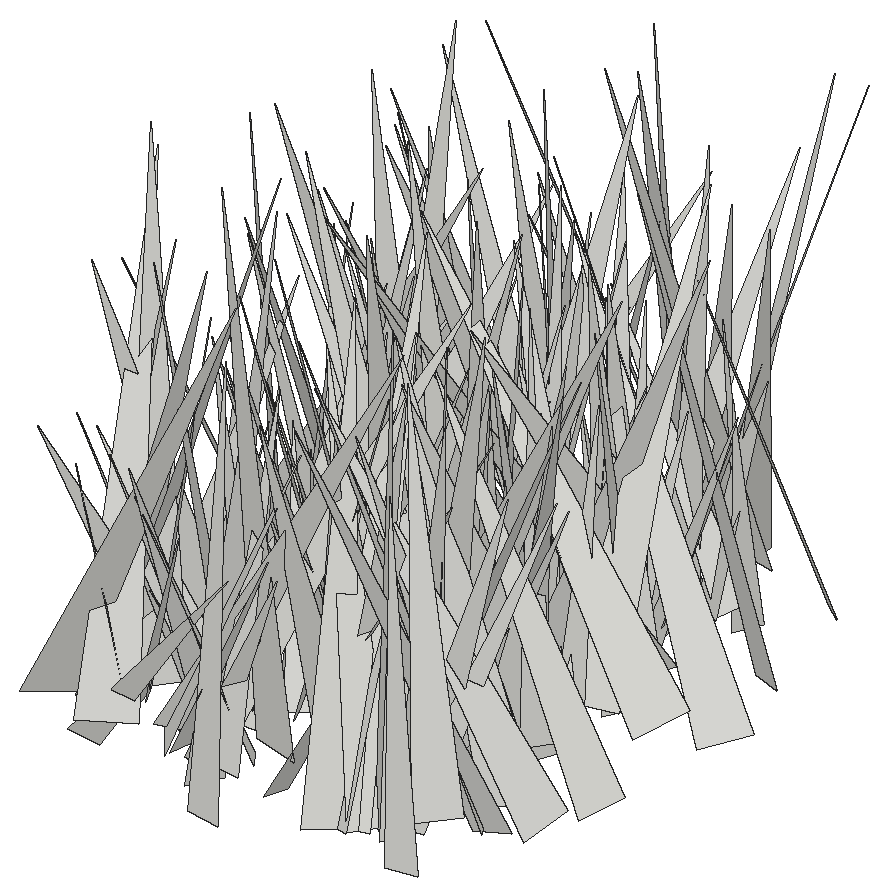
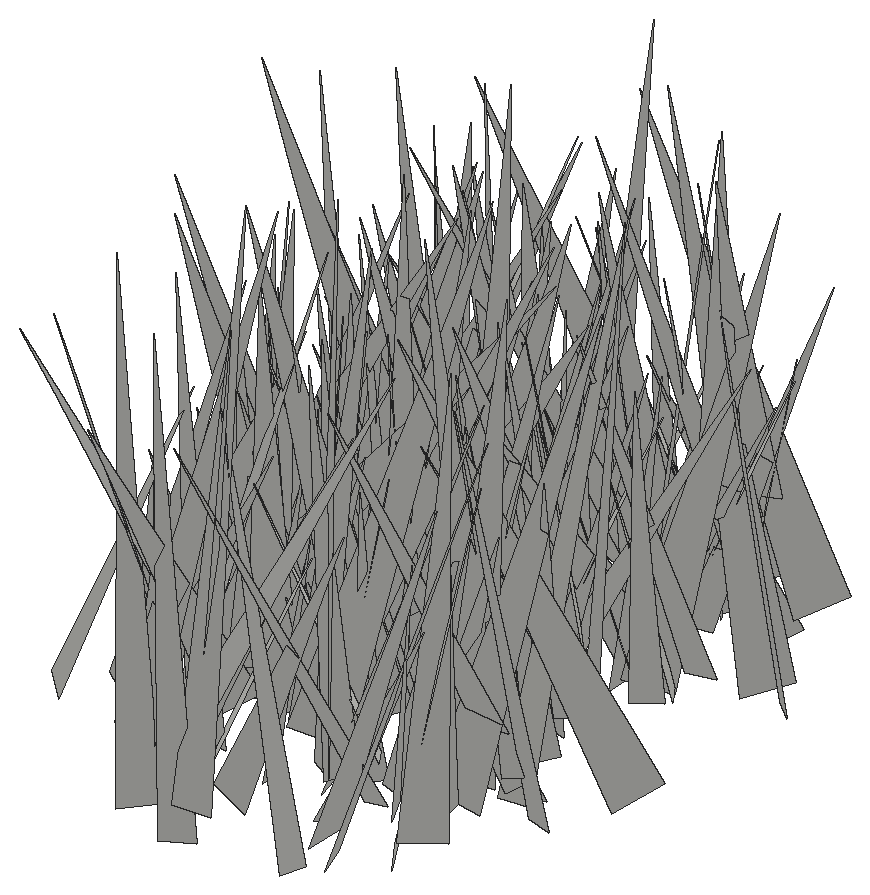
# SketchUp Ruby script. Lengths in inches.
U = 1.inch
M = Sketchup.active_model
def pt(a) = Geom::Point3d.new(a.map { |v| v * U })
def face(e, loops, mat)
  f = e.add_face(loops[0].map { |a| pt(a) })
  loops[1..].each { |l| e.add_face(l.map { |a| pt(a) }).erase! }
  f.material = f.back_material = mat if mat
  f
end
# faces: each face lists its corners as indices into pts; further lists are holes
def faces(e, pts, list, mat = nil) = list.each { |f| face(e, (f[0].is_a?(Array) ? f : [f]).map { |l| l.map { |i| pts[i] } }, mat) }
# xy, xz, yz: faces in a plane at the given z, y or x. An outline is a flat list of corners, or four numbers for a rectangle; further outlines are holes
def ring(l) = l.size == 4 ? [[l[0], l[1]], [l[2], l[1]], [l[2], l[3]], [l[0], l[3]]] : l.each_slice(2).to_a
def flat(e, list, mat, &to3) = list.each { |f| face(e, (f[0].is_a?(Array) ? f : [f]).map { |l| ring(l).map { |u, v| to3.(u, v) } }, mat) }
def xy(e, z, list, mat = nil) = flat(e, list, mat) { |x, y| [x, y, z] }
def xz(e, y, list, mat = nil) = flat(e, list, mat) { |x, z| [x, y, z] }
def yz(e, x, list, mat = nil) = flat(e, list, mat) { |y, z| [x, y, z] }
def lines(e, pts, list) = list.each { |a, b| e.add_line(pt(pts[a]), pt(pts[b])) }
# prism: a flat outline (further loops are holes) pulled along v
def prism(e, loops, v, mat = nil)
  f = face(e, loops, mat); d = Geom::Vector3d.new(v.map { |x| x * U })
  f.pushpull(f.normal.samedirection?(d) ? d.length : -d.length)
end
def box(e, o, s, mat = nil) = prism(e, [[o, [o[0] + s[0], o[1], o[2]], [o[0] + s[0], o[1] + s[1], o[2]], [o[0], o[1] + s[1], o[2]]]], [0, 0, s[2]], mat)
def at(x, y, z, deg = 0) = Geom::Transformation.translation(pt([x, y, z])) * Geom::Transformation.rotation(ORIGIN, Z_AXIS, deg.degrees)
def axes(o, x, y, z) = Geom::Transformation.new([*x, 0, *y, 0, *z, 0, *pt(o).to_a, 1])
def part(name) = M.definitions.add(name)
# library, detail: a bought-in or finely detailed component or shape, given as its bounding box
def library(name, o, s) = part(name).tap { |d| box(d.entities, o, s) }
def detail(e, o, s) = box(e.add_group.entities, o, s)
def put(e, d, t, mat = nil) = e.add_instance(d, t).tap { |i| i.material = mat if mat }
def group(e, t, mat = nil) = e.add_group.tap { |g| g.transformation = t; g.material = mat if mat }.entities
root = M.entities
c1 = part("fur_instance\#9")
p = [[0.8125,0,1.79],[0.67,-0.02,1.48],[0,-0.11,0],[0,0.11,0]]
faces(c1.entities,p,[[0,1,2,3]])
put(root,c1,axes([110.54,92.22,-28.22],[5.37674,4.78999,2.15375],[5.23773,-5.117,-1.69543],[-0.38579,-2.71372,6.99849]))
put(root,c1,axes([113.62,104.89,-28.22],[-4.7875,-3.33897,1.34753],[-3.4677,4.87923,-0.23006],[0.96934,0.96392,5.83232]))
put(root,c1,axes([114.25,101.53,-28.22],[0.14854,-7.36709,1.66817],[-7.40985,-0.46607,-1.39849],[-1.46661,1.60862,7.23466]))
put(root,c1,axes([112.35,95.74,-27.1],[2.0816,-3.74764,1.04429],[-3.88491,-2.06538,0.3318],[-0.20701,1.076,4.27408]))
put(root,c1,axes([111.72,101.13,-28.22],[3.01267,4.99828,1.819],[5.31773,-2.78497,-1.15474],[0.11548,-2.15148,5.72063]))
put(root,c1,axes([114.11,88.5,-27.1],[-5.29033,5.65073,1.03717],[5.57546,5.38985,-0.92613],[1.38587,-0.11308,7.68509]))
put(root,c1,axes([116.16,95.35,-28.22],[-3.99389,-5.07881,0.29207],[-4.86869,3.70838,-2.09153],[-1.47493,1.51142,6.11318]))
put(root,c1,axes([114.78,106.07,-28.22],[-6.09562,-2.74651,0.83103],[-2.67616,6.14538,0.68045],[1.03541,-0.28555,6.65108]))
put(root,c1,axes([114.16,93.5,-28.22],[3.31279,-6.01066,2.01721],[-5.81791,-3.7865,-1.72802],[-2.51972,0.84034,6.64203]))
put(root,c1,axes([112.27,105.35,-27.1],[4.76035,-4.27512,0.72339],[-4.20428,-4.81383,-0.78223],[-1.06017,-0.10597,6.35025]))
put(root,c1,axes([115.68,105.08,-28.22],[-6.67851,0.63047,0.27765],[0.60623,6.66388,-0.54986],[0.32721,0.52189,6.68563]))
put(root,c1,axes([113.89,90.8,-27.1],[5.91163,-3.56463,4.13587],[-4.286,-6.80601,0.26026],[-3.38262,2.39395,6.89828]))
put(root,c1,axes([114.8,91.125,-27.1],[-3.58425,-2.16039,0.18109],[-2.16614,3.55434,-0.47063],[-0.08907,0.49634,4.15845]))
put(root,c1,axes([113.89,104.45,-27.1],[-3.72029,-1.54775,1.40082],[-1.82397,3.80239,-0.64288],[1.01535,1.15959,3.97778]))
put(root,c1,axes([113.86,91.77,-27.1],[3.91388,-2.85851,1.41513],[-2.09693,-3.9939,-2.26798],[-2.40345,-1.17037,4.2832]))
put(root,c1,axes([113.86,89.69,-27.1],[2.36967,1.89121,2.13493],[2.35412,-2.86396,-0.07595],[-1.61018,-1.40392,3.03088]))
put(root,c1,axes([112.15,93.71,-27.1],[0.82135,5.31818,1.14764],[5.3338,-0.55827,-1.23031],[1.07271,-1.29616,5.2387]))
put(root,c1,axes([114.93,96.82,-28.22],[-0.43332,5.55714,0.38235],[5.39105,0.32188,1.43136],[-1.40165,-0.47995,5.3871]))
put(root,c1,axes([115.21,92.45,-28.22],[-4.40105,0.97982,0.44244],[1.06612,4.21791,1.26401],[0.13855,-1.33202,4.328]))
put(root,c1,axes([110.55,98.36,-28.22],[6.56364,-3.25708,1.01889],[-3.38805,-5.95385,2.79299],[0.40967,2.94467,6.77415]))
put(root,c1,axes([114.24,95.81,-28.22],[-4.94486,-5.49387,2.91837],[-6.02867,5.15162,-0.51692],[1.53451,2.53562,7.37341]))
put(root,c1,axes([113.36,93.34,-28.22],[2.95559,2.2846,0.71516],[2.24296,-3.03986,0.44126],[-0.83663,-0.07885,3.70947]))
put(root,c1,axes([112.98,100.57,-28.22],[-2.73458,-7.67612,0.26637],[-7.34259,2.69559,2.30041],[2.25392,-0.53168,7.81722]))
put(root,c1,axes([112.49,101.03,-27.1],[0.76926,-4.66703,1.07076],[-4.59745,-0.41678,1.48633],[1.33832,1.25083,4.49041]))
put(root,c1,axes([111.45,97.96,-28.22],[2.70061,4.81345,0.08968],[4.52857,-2.505,-1.92033],[1.63383,-1.01307,5.17446]))
put(root,c1,axes([114.73,100.41,-28.22],[1.15068,-6.84996,3.27998],[-7.48842,-1.57649,-0.66528],[-1.26644,3.09791,6.914]))
put(root,c1,axes([114.79,93.77,-28.22],[-4.88413,-0.13594,1.40409],[-0.16648,5.08029,-0.08723],[1.4008,0.12978,4.88524]))
put(root,c1,axes([113.99,102.03,-28.22],[3.8396,0.83392,1.68617],[0.96833,-4.16197,-0.14664],[-1.61273,-0.51356,3.92638]))
put(root,c1,axes([114.99,100.08,-28.22],[-4.38014,-2.49103,0.91186],[-2.44951,4.47381,0.4553],[1.01814,0.04674,5.01832]))
put(root,c1,axes([111.52,91.66,-28.22],[8.0282,-2.33719,0.44231],[-2.30718,-8.02996,-0.55383],[-0.57877,-0.40914,8.34313]))
put(root,c1,axes([114.03,90.35,-27.1],[4.42151,2.80893,1.55928],[2.73673,-4.68252,0.67492],[-1.68278,-0.23477,5.19464]))
put(root,c1,axes([116.12,104.46,-28.22],[-3.16167,2.60611,0.16715],[2.5519,3.02748,1.0668],[-0.55458,-0.92652,3.956]))
put(root,c1,axes([112.67,90.4,-27.1],[7.43833,2.19546,1.23858],[2.06036,-7.51855,0.95355],[-1.45225,0.57818,7.69672]))
put(root,c1,axes([115.7,100.08,-27.1],[-3.05082,2.35934,0.28628],[2.37608,3.01778,0.45074],[-0.05159,-0.53147,3.83025]))
put(root,c1,axes([116.54,94.38,-27.1],[-4.07706,-2.14403,0.24298],[-2.12817,3.90987,-1.20919],[-0.35608,1.18084,4.44491]))
put(root,c1,axes([115.99,99.75,-28.22],[-4.01169,-3.78695,1.3287],[-4.00574,3.89344,-0.9976],[0.2459,1.64323,5.42581]))
put(root,c1,axes([115.84,90.8125,-27.1],[-3.47734,-1.80435,0.22841],[-1.8088,3.48242,-0.02761],[0.19,0.12974,3.9175]))
put(root,c1,axes([114.99,94.75,-28.22],[4.45887,4.52554,1.75159],[4.30275,-4.78695,1.41478],[-2.24387,-0.18639,6.19358]))
put(root,c1,axes([112.76,100.27,-28.22],[0.65701,6.39206,0.99008],[6.12037,-0.29236,-2.17392],[2.09278,-1.15171,6.04683]))
put(root,c1,axes([114.97,100.19,-27.1],[-4.71927,-1.33587,1.95814],[-1.09743,5.09822,0.83318],[2.10107,-0.33763,4.83341]))
put(root,c1,axes([113.78,98.33,-28.22],[3.6262,-2.26105,0.60128],[-2.31235,-3.63241,0.28605],[-0.35624,0.56255,4.26378]))
put(root,c1,axes([114.69,99.76,-27.1],[0.76042,7.54721,2.45249],[7.93568,-0.724,-0.23253],[-0.00259,-2.46349,7.58186]))
put(root,c1,axes([111.92,88.86,-27.1],[6.68383,-3.60485,0.36068],[-3.59385,-6.50181,1.61538],[0.45749,1.59067,7.42019]))
put(root,c1,axes([116.02,95.29,-28.22],[-1.82389,-4.57282,0.8897],[-4.65371,1.74485,-0.5721],[-0.21262,1.03617,4.88978]))
put(root,c1,axes([113.45,97.68,-27.1],[0.14432,-5.01914,1.5992],[-4.96199,0.40759,1.72702],[1.76858,1.55311,4.71487]))
put(root,c1,axes([115.32,92.33,-28.22],[-6.01698,-4.0059,2.23214],[-3.85326,6.41302,1.12219],[2.48637,0.24439,7.14087]))
put(root,c1,axes([117.45,102.66,-28.22],[-6.60705,-1.5953,0.55499],[-1.61141,6.62494,-0.14037],[0.50631,0.26714,6.79547]))
put(root,c1,axes([115.55,92.09,-28.22],[-4.95607,3.58078,0.35964],[3.00453,4.45388,-2.94106],[1.98095,2.2034,5.36049]))
put(root,c1,axes([117.55,94.45,-27.1],[-2.16703,-5.16397,2.37315],[-5.48971,1.24499,-2.30381],[-1.47021,2.96275,5.10441]))
put(root,c1,axes([116.35,99.25,-28.22],[-6.49711,1.14641,2.18071],[1.63194,6.61021,1.38712],[1.84567,-1.80917,6.45001]))
put(root,c1,axes([115.87,102.11,-28.22],[-1.28236,-4.10189,0.60594],[-4.14572,1.27987,-0.10961],[0.07509,0.61118,4.29626]))
put(root,c1,axes([112.89,89.08,-28.22],[2.58418,-3.37784,0.00054],[-2.92311,-2.23595,2.1316],[1.69269,1.29557,3.68023]))
put(root,c1,axes([114.99,98.35,-28.22],[2.68413,-2.59886,0.79499],[-2.66781,-2.73276,0.07385],[-0.51851,0.60713,3.7354]))
put(root,c1,axes([114.16,89.83,-27.1],[3.91302,0.34843,0.25725],[0.41449,-3.69091,-1.30566],[-0.12562,-1.32482,3.70519]))
put(root,c1,axes([115.92,90.53,-27.1],[0.4513,-4.46287,0.47479],[-4.46772,-0.49211,-0.3789],[-0.42669,0.43236,4.4696]))
put(root,c1,axes([115.26,98.74,-27.1],[2.93725,2.51058,1.33666],[2.80043,-2.8887,-0.72813],[-0.49727,-1.43859,3.79478]))
put(root,c1,axes([117.31,95.83,-27.1],[2.82941,3.82153,3.56935],[4.50896,-3.83832,0.53527],[-2.64833,-2.45217,4.72474]))
put(root,c1,axes([115.95,96.2,-27.1],[2.7326,-2.75522,2.01665],[-3.2693,-2.85632,0.52755],[-0.98478,1.83723,3.84448]))
put(root,c1,axes([115.56,99.15,-27.1],[2.99735,3.72962,0.28981],[3.68324,-3.00724,0.60693],[-0.65404,0.15682,4.74613]))
put(root,c1,axes([116.83,89.17,-28.22],[-7.30658,0.78889,2.52937],[0.00726,7.42557,-2.29501],[2.64953,2.15518,6.98151]))
put(root,c1,axes([116.79,93.56,-27.1],[-6.46453,1.71895,1.7422],[0.79023,6.12289,-3.109],[2.31637,2.70842,5.92275]))
put(root,c1,axes([118.99,105.15,-28.22],[-0.49335,5.1966,1.87912],[5.02115,-0.36617,2.33091],[-2.30734,-1.90798,4.67065]))
put(root,c1,axes([116.36,96.8,-27.1],[4.45017,0.43948,1.54669],[0.28501,-4.6951,0.51402],[-1.58245,0.39027,4.44218]))
put(root,c1,axes([118.32,89.36,-27.1],[-3.2308,-2.41105,0.08917],[-2.40238,3.20101,-0.49122],[-0.22293,0.4467,4.00124]))
put(root,c1,axes([117.72,92.03,-27.1],[-2.46678,3.0111,0.36551],[3.02886,2.4705,0.08915],[0.1623,-0.33942,3.8915]))
put(root,c1,axes([117.37,92.78,-27.1],[1.88548,3.67223,0.79609],[3.49899,-2.04056,1.12569],[-1.36969,-0.15771,3.97154]))
put(root,c1,axes([115.9,91.76,-27.1],[-0.80392,-5.00028,1.94874],[-5.12712,1.2977,1.21465],[1.58527,1.66129,4.91668]))
put(root,c1,axes([114.54,104.47,-27.1],[2.28513,5.39499,0.34939],[5.12885,-2.04337,-1.99232],[1.70965,-1.08097,5.50984]))
put(root,c1,axes([115.28,92.85,-28.22],[3.56732,3.05528,0.6125],[3.0981,-3.37772,-1.19517],[0.33415,-1.30074,4.54225]))
put(root,c1,axes([119.83,95.01,-28.22],[-2.53782,7.33959,2.16761],[7.45924,1.86167,2.42953],[-1.71111,-2.77006,7.37615]))
put(root,c1,axes([118,102.64,-27.1],[3.07442,-7.15508,0.96712],[-6.88437,-3.22185,-1.95131],[-2.1762,0.08396,7.5392]))
put(root,c1,axes([115.79,98.77,-28.22],[3.45367,-2.54495,0.42724],[-2.57712,-3.36456,0.79082],[0.1334,0.88889,4.21654]))
put(root,c1,axes([121.15,105.39,-28.22],[-6.03257,-5.76703,0.56772],[-5.59645,5.58532,-2.7307],[-1.50355,2.34912,7.8863]))
put(root,c1,axes([118.68,93.71,-27.1],[-2.89225,-3.68575,0.79235],[-3.76683,2.78458,-0.79678],[-0.15371,1.11313,4.61682]))
put(root,c1,axes([118.02,87.6,-28.22],[1.54209,5.92638,1.72605],[6.04197,-1.81335,0.82809],[-1.2633,-1.43843,6.06748]))
put(root,c1,axes([115.24,107.13,-28.22],[6.27835,0.76334,0.54412],[0.88551,-6.03847,-1.74618],[-0.30762,-1.80294,6.07875]))
put(root,c1,axes([116.19,103.89,-27.1],[5.48101,-1.25937,0.85366],[-1.15676,-5.52263,-0.72019],[-0.98826,-0.52035,5.57753]))
put(root,c1,axes([118.89,93.01,-27.1],[-4.07714,-4.72232,1.18622],[-4.85623,4.056,-0.54439],[0.3528,1.25658,6.21506]))
put(root,c1,axes([119.25,92.47,-27.1],[-2.70694,-4.99144,1.16007],[-5.08628,2.45713,-1.29614],[-0.62448,1.62351,5.52829]))
put(root,c1,axes([120.14,100.26,-28.22],[-1.35129,-7.71927,0.81651],[-7.46816,1.06686,-2.27338],[-2.11671,1.16382,7.49966]))
put(root,c1,axes([121.85,94.5,-28.22],[-2.8355,7.09509,0.7949],[6.33308,2.10473,3.80453],[-3.2961,-2.05963,6.62616]))
put(root,c1,axes([116.03,102.46,-27.1],[3.45283,2.51437,0.03768],[2.48973,-3.40925,-0.65094],[0.3531,-0.54815,4.22141]))
put(root,c1,axes([115.59,96.75,-28.22],[4.52674,3.32324,0.78926],[3.39525,-4.2348,-1.64226],[0.37301,-1.78348,5.37013]))
put(root,c1,axes([118.47,90.05,-27.1],[-2.90002,-7.26429,3.03178],[-7.85451,2.88308,-0.60516],[0.51793,3.0479,7.79832]))
put(root,c1,axes([118.07,100.4,-28.22],[-3.76859,1.24193,1.36163],[1.17189,4.00702,-0.41131],[1.42236,-0.01087,3.94658]))
put(root,c1,axes([117.35,93.17,-27.1],[-1.65671,-3.63214,1.3485],[-3.6613,1.94738,0.7471],[1.26719,0.87797,3.92161]))
put(root,c1,axes([115.96,88.61,-27.1],[4.04604,3.23344,0.3968],[3.2461,-3.94826,-0.92578],[0.27467,-0.96906,5.09593]))
put(root,c1,axes([116.8,103.95,-27.1],[-4.19902,-6.23031,2.61813],[-6.01537,4.8505,1.89504],[3.08005,0.97931,7.27031]))
put(root,c1,axes([118.91,97.6,-28.22],[-7.37907,1.498,2.27835],[1.63074,7.6926,0.22378],[2.18531,-0.6822,7.52626]))
put(root,c1,axes([116.47,88.63,-27.1],[3.59656,-0.31618,0.04156],[-0.31764,-3.59357,0.14939],[-0.02828,0.15246,3.60734]))
put(root,c1,axes([118.05,88.39,-27.1],[0.83118,5.18677,1.07004],[5.28228,-0.88982,0.21009],[-0.38088,-1.02179,5.24874]))
put(root,c1,axes([120.16,96.15,-28.22],[-6.63907,0.80935,0.83748],[0.8673,6.67065,0.42894],[0.7773,-0.53025,6.67446]))
put(root,c1,axes([116.25,89.71,-28.22],[1.31964,-4.20384,0.49444],[-3.9297,-1.02429,1.77946],[1.57296,0.96785,4.03079]))
put(root,c1,axes([118.99,100.53,-28.22],[-3.57369,-1.9669,1.0397],[-2.0892,3.64317,-0.28897],[0.76478,0.76131,4.06896]))
put(root,c1,axes([116.59,102.02,-28.22],[1.3305,-3.93215,0.09517],[-3.71952,-1.22514,1.38031],[1.27907,0.52755,3.91494]))
put(root,c1,axes([118.8125,101.97,-27.1],[-6.63003,0.58928,2.6026],[0.94805,7.03587,0.82207],[2.49439,-1.10786,6.6052]))
put(root,c1,axes([118.83,103.61,-28.22],[-3.35519,-0.75879,1.11745],[-0.66434,3.53232,0.40387],[1.17606,-0.1694,3.41613]))
put(root,c1,axes([118.22,94.5,-28.22],[4.04472,-2.80495,1.23292],[-2.68281,-4.22845,-0.81868],[-1.47998,-0.00072,4.85358]))
put(root,c1,axes([117.53,96.41,-27.1],[7.0973,-2.99001,1.53723],[-2.6894,-7.20395,-1.59536],[-2.01752,-0.91535,7.53436]))
put(root,c1,axes([115.54,90.43,-28.22],[1.59933,7.72158,1.03232],[7.26868,-1.09996,-3.03359],[2.80263,-1.55359,7.2786]))
put(root,c1,axes([119.64,92.17,-28.22],[-5.27031,-0.93158,1.82448],[-1.52104,5.15288,-1.7627],[1.37223,2.13373,5.05341]))
put(root,c1,axes([119.65,105.53,-27.1],[-6.31517,-2.67121,2.41272],[-3.08957,6.52254,-0.86542],[1.84694,1.77736,6.80204]))
put(root,c1,axes([117.92,93.19,-28.22],[5.02867,-2.50397,0.95955],[-2.41233,-5.11484,-0.70513],[-1.17101,-0.21602,5.57317]))
put(root,c1,axes([118.32,98.19,-28.22],[2.03381,4.83721,0.83738],[4.90479,-2.04045,-0.1258],[-0.20703,-0.82108,5.24587]))
put(root,c1,axes([121.31,104.45,-28.22],[-2.97,-5.19915,0.68344],[-5.09037,2.66981,-1.8109],[-1.25951,1.46972,5.70725]))
put(root,c1,axes([119.75,100.43,-27.1],[4.32475,3.25099,2.86901],[3.37923,-5.06616,0.64681],[-2.71679,-1.12634,5.37159]))
put(root,c1,axes([119.16,91.7,-27.1],[1.67149,-5.33301,0.8085],[-5.34441,-1.75188,-0.5067],[-0.72935,0.6152,5.5658]))
put(root,c1,axes([120.9,103.34,-28.22],[-3.56795,-1.90054,0.20659],[-1.88749,3.43261,-1.0196],[-0.30353,0.99505,3.91187]))
put(root,c1,axes([117.57,92.26,-27.1],[5.27684,1.71083,0.85913],[1.8324,-5.24307,-0.81398],[-0.55438,-1.04563,5.4872]))
put(root,c1,axes([115.9375,89.38,-27.1],[5.9864,-4.39629,0.74457],[-4.35138,-5.48795,2.58196],[0.97326,2.50473,6.96403]))
put(root,c1,axes([118.77,97.91,-27.1],[2.85129,3.39796,1.84964],[3.79237,-2.9092,-0.50161],[-0.76499,-1.75715,4.40731]))
put(root,c1,axes([118.12,107.84,-27.1],[-1.88375,-7.99896,1.23534],[-7.80751,2.13018,1.88761],[2.13359,0.73274,7.99805]))
put(root,c1,axes([118.39,98.65,-28.22],[7.00851,-2.19777,2.01204],[-2.01969,-7.2848,-0.92211],[-2.19075,-0.31499,7.28692]))
put(root,c1,axes([123.64,99.57,-27.1],[-2.19661,-7.3796,0.4517],[-6.30745,1.62463,-4.13089],[-3.85727,1.54587,6.49764]))
put(root,c1,axes([120.54,100.48,-28.22],[-2.76713,3.18046,1.2921],[3.43249,2.58898,0.97827],[0.05304,-1.61979,4.10065]))
put(root,c1,axes([120.65,98.42,-27.1],[0.64289,6.12986,1.03372],[6.0316,-0.86662,1.38779],[-1.50455,-0.85491,6.00521]))
put(root,c1,axes([118.69,95.09,-27.1],[6.30569,-0.68619,2.05979],[-1.17683,-6.39727,1.4715],[-1.82446,1.75482,6.16987]))
put(root,c1,axes([118.48,99.68,-27.1],[-2.56408,6.91655,2.55207],[6.94878,3.17004,-1.60986],[2.46298,-1.74312,7.19872]))
put(root,c1,axes([119.12,92.14,-27.1],[3.9195,-3.82723,2.46639],[-4.43668,-3.94163,0.93419],[-1.02305,2.43088,5.39791]))
put(root,c1,axes([120.93,89.24,-28.22],[-5.83364,4.02968,1.05878],[3.90844,5.92385,-1.01134],[1.44341,0.24573,7.01761]))
put(root,c1,axes([121.55,98.9,-28.22],[-3.34146,5.15286,1.47209],[5.35695,3.16362,1.08579],[-0.14849,-1.82317,6.0447]))
put(root,c1,axes([121.8,89.95,-28.22],[-5.57386,3.34507,0.61319],[3.34749,5.6042,-0.14346],[0.5998,-0.19191,6.49898]))
put(root,c1,axes([121.06,89.49,-28.22],[-1.39232,7.88876,0.40308],[7.89477,1.37627,0.33483],[-0.26016,-0.45487,8.00369]))
put(root,c1,axes([121.25,97.19,-27.1],[-5.97598,0.81352,1.54005],[0.17172,5.75229,-2.37225],[1.73323,2.235,5.54496]))
put(root,c1,axes([120.46,97.49,-28.22],[-3.28983,-1.54802,1.9149],[-2.00034,3.5437,-0.57187],[1.43591,1.38997,3.59058]))
put(root,c1,axes([118.62,107.8,-28.22],[-0.2881,-6.79413,1.19024],[-6.52945,0.65262,2.14482],[2.22333,1.03623,6.45314]))
put(root,c1,axes([122.03,103.33,-27.1],[-4.79453,-5.10071,1.01007],[-5.15614,4.84133,-0.02673],[0.67211,0.75447,7.00029]))
put(root,c1,axes([121.81,105.67,-27.1],[-2.25691,-7.5793,1.44794],[-7.71352,2.17504,-0.63772],[-0.20948,1.56823,7.88243]))
put(root,c1,axes([118.64,89.85,-28.22],[5.85572,0.96623,0.0245],[0.91904,-5.61274,1.69591],[-0.29926,1.66948,5.68743]))
put(root,c1,axes([119.875,91.41,-28.22],[5.45486,-2.53583,1.72286],[-2.73109,-5.61705,0.37948],[-1.39279,1.08278,6.00349]))
put(root,c1,axes([121.38,100.27,-28.22],[-2.53684,6.34204,1.9532],[6.60869,2.60398,0.12835],[0.60133,-1.86275,6.82939]))
put(root,c1,axes([119.32,99.12,-27.1],[4.77577,-2.2799,0.31782],[-2.26651,-4.78515,-0.26858],[-0.40236,-0.10607,5.28524]))
put(root,c1,axes([120.71,102.58,-27.1],[-4.56425,4.1816,0.8559],[3.58274,4.43445,-2.55936],[2.31998,1.37862,5.63629]))
put(root,c1,axes([121.05,96.11,-28.22],[4.35483,5.04158,0.80125],[4.65214,-4.35304,2.10539],[-2.1017,0.81089,6.32055]))
put(root,c1,axes([120.5,99.71,-28.22],[3.85883,-1.0172,1.02296],[-0.87371,-3.97244,-0.65425],[-1.14794,-0.39587,3.93665]))
put(root,c1,axes([121.1,89.375,-28.22],[1.43263,3.39143,0.32506],[3.34277,-1.46736,0.57677],[-0.65831,-0.07043,3.63615]))
put(root,c1,axes([123.1,103.3,-27.1],[-4.21656,2.08304,0.19454],[2.06998,4.09043,1.06765],[-0.30342,-1.04195,4.58024]))
put(root,c1,axes([121.26,95.42,-28.22],[-5.60874,-1.91132,2.91151],[-2.48414,6.06379,-0.80475],[2.44113,1.77916,5.87056]))
put(root,c1,axes([119.71,100.33,-27.1],[4.16125,-1.09144,0.28201],[-1.11074,-4.15389,0.31328],[-0.19241,0.37504,4.29058]))
put(root,c1,axes([121.36,97.18,-27.1],[-1.65824,-4.82946,1.36253],[-4.95542,1.80194,0.35604],[0.78993,1.16588,5.09379]))
put(root,c1,axes([122.86,98.57,-28.22],[-4.31173,0.11749,0.33288],[0.02447,4.16916,-1.1546],[0.35215,1.14887,4.15592]))
put(root,c1,axes([123.82,92.02,-28.22],[-5.99234,-4.15881,0.58341],[-4.19764,5.96205,-0.6148],[0.12593,0.83815,7.26814]))
put(root,c1,axes([121.08,99.9,-27.1],[4.15437,2.45212,1.76514],[2.75663,-4.30471,-0.50784],[-1.23677,-1.35794,4.79727]))
put(root,c1,axes([121.47,103,-28.22],[-1.17344,-6.36654,3.3674],[-7.15717,1.41187,0.17527],[0.80444,3.27459,6.4714]))
put(root,c1,axes([122.27,93.22,-27.1],[-5.24413,-0.63684,1.6828],[-0.10679,5.28634,1.66778],[1.7961,-1.54509,5.01248]))
put(root,c1,axes([125.45,97.34,-27.1],[-6.72983,3.60579,0.05795],[3.45053,6.40273,2.3226],[-1.04828,-2.07339,7.27309]))
put(root,c1,axes([120.54,93.52,-28.22],[0.4901,-6.09421,1.40714],[-6.12992,-0.18765,1.32232],[1.24239,1.47818,5.96918]))
put(root,c1,axes([121.23,97.07,-27.1],[-1.26744,-3.38882,1.28492],[-3.35573,1.6115,0.94004],[1.36901,0.81271,3.49382]))
put(root,c1,axes([122.45,101.63,-27.1],[6.08199,-2.63161,2.26399],[-1.13407,-5.82276,-3.72169],[-3.281,-2.8656,5.48316]))
put(root,c1,axes([122.45,104.57,-27.1],[0.90627,3.33198,1.59944],[3.57947,-1.20149,0.47479],[-0.9207,-1.39138,3.42023]))
put(root,c1,axes([122.21,89.8,-28.22],[4.06784,5.47307,2.7985],[5.78633,-4.54195,0.47187],[-2.07475,-1.93641,6.80288]))
put(root,c1,axes([123.79,93.14,-28.22],[2.26565,-5.57265,3.25786],[-5.77256,-3.29433,-1.62055],[-2.88887,2.21229,5.79322]))
put(root,c1,axes([123.61,94.45,-27.1],[-5.70107,0.73605,0.76728],[0.48907,5.53142,-1.67238],[0.94409,1.57933,5.49974]))
put(root,c1,axes([121.75,100.14,-27.1],[1.49133,-6.04191,1.54576],[-6.23212,-1.50337,0.13646],[-0.23383,1.53405,6.22175]))
put(root,c1,axes([121.93,92.33,-28.22],[4.77754,4.17311,2.72058],[4.61145,-5.13068,-0.22808],[-1.8844,-1.97551,6.33938]))
put(root,c1,axes([123.04,96.03,-28.22],[3.93068,-5.30389,1.53813],[-4.85639,-4.21869,-2.1367],[-2.62918,-0.13704,6.24628]))
put(root,c1,axes([121.75,100.75,-27.1],[4.45698,-3.93649,1.376],[-3.92382,-4.64074,-0.56675],[-1.41173,0.47074,5.91941]))
put(root,c1,axes([125.21,92.83,-28.22],[-6.69596,1.51903,0.23584],[1.52209,6.40398,1.96756],[-0.2152,-1.96993,6.57815]))
put(root,c1,axes([120.66,93.9375,-27.1],[0.32033,-6.88611,1.90206],[-6.92731,0.16595,1.76741],[1.74605,1.92169,6.66313]))
put(root,c1,axes([124.32,91.74,-28.22],[-0.7364,-6.55979,0.93298],[-6.36781,0.44127,-1.92351],[-1.83094,1.10364,6.31453]))
put(root,c1,axes([122.46,99.18,-28.22],[-2.24525,-3.81491,0.32062],[-3.67914,2.25292,1.04201],[1.05843,-0.26136,4.3022]))
put(root,c1,axes([122.625,89.85,-28.22],[-2.66914,2.15187,1.53787],[2.38339,2.90414,0.07299],[1.14676,-1.02728,3.42776]))
put(root,c1,axes([121.25,94.05,-28.22],[3.95352,-1.35205,0.74696],[-1.51739,-3.78343,1.18299],[-0.28899,1.3689,4.00736]))
put(root,c1,axes([122.62,102.74,-27.1],[3.92721,6.27569,0.86047],[6.07775,-4.01843,1.56873],[-1.78486,0.12492,7.23508]))
put(root,c1,axes([122.84,99.28,-27.1],[-0.37436,4.96388,1.61425],[5.21969,0.34743,0.14211],[-0.02763,-1.62026,4.97594]))
put(root,c1,axes([123.27,99.22,-28.22],[-3.51075,4.42455,2.16586],[4.8357,3.60279,0.47842],[0.94002,-2.00904,5.62789]))
put(root,c1,axes([122.1875,101.59,-27.1],[6.2923,4.31715,0.79405],[3.75537,-6.01297,2.93303],[-2.27277,2.01685,7.04472]))
put(root,c1,axes([120.64,106.9375,-28.22],[7.2919,-1.58164,0.56037],[-1.39543,-7.10365,-1.89164],[-0.93186,-1.73896,7.21769]))
put(root,c1,axes([122.06,99.75,-28.22],[0.83525,-3.69964,2.10924],[-4.22949,-0.46947,0.8514],[0.49764,2.21949,3.69595]))
put(root,c1,axes([121.68,96.46,-27.1],[4.68677,-2.0034,0.66372],[-1.95488,-4.73014,-0.47351],[-0.79535,-0.17932,5.07496]))
put(root,c1,axes([126.06,99.23,-28.22],[-4.44973,5.42889,0.1833],[5.21151,4.19987,2.12315],[-1.53186,-1.48148,6.69068]))
put(root,c1,axes([119.4,95.34,-27.1],[5.85705,-5.48153,0.51052],[-5.36351,-5.5136,2.33363],[1.24121,2.04104,7.67505]))
put(root,c1,axes([122.89,96.6,-28.22],[0.37459,4.6587,1.44665],[4.87681,-0.39143,-0.00226],[-0.11359,-1.44218,4.67373]))
put(root,c1,axes([124.92,102.36,-28.22],[-3.81075,-5.76969,1.72606],[-6.01138,3.52106,-1.50194],[-0.36316,2.25903,6.74947]))
put(root,c1,axes([120.625,98.16,-28.22],[6.76451,-3.26106,1.25254],[-3.47694,-6.54929,1.72622],[-0.33809,2.1058,7.30844]))
put(root,c1,axes([122.17,100.46,-28.22],[3.86814,-0.78573,1.02615],[-1.07279,-3.75781,1.16655],[-0.72076,1.37634,3.77081]))
put(root,c1,axes([122.77,104.28,-28.22],[3.12862,-2.29976,0.97047],[-2.27,-3.26853,-0.42753],[-1.03819,0.21622,3.85932]))
put(root,c1,axes([123.78,88.63,-28.22],[-0.00345,4.9845,1.60202],[5.18158,-0.22632,0.71534],[-0.75028,-1.58596,4.93291]))
put(root,c1,axes([122.34,100.08,-28.22],[5.99792,1.55177,2.60045],[2.40829,-5.94226,-2.00876],[-1.83589,-2.72525,5.86071]))
put(root,c1,axes([121.25,92.625,-27.1],[6.06997,0.80019,0.53139],[0.73411,-6.05703,0.73529],[-0.61948,0.66277,6.07817]))
put(root,c1,axes([125.77,94.46,-28.22],[-6.12139,2.10353,0.29479],[2.12072,6.0019,1.20952],[-0.1196,-1.23917,6.35872]))
put(root,c1,axes([124.07,89.79,-27.1],[-4.47005,3.93119,1.60818],[4.11701,4.5843,0.23722],[1.04438,-1.24571,5.94805]))
put(root,c1,axes([121.75,91.83,-28.22],[-0.77614,4.62516,2.62163],[4.88719,1.66369,-1.48826],[2.09294,-2.16967,4.44742]))
put(root,c1,axes([125.21,104.75,-27.1],[-3.55918,-3.90599,0.48478],[-3.91702,3.45103,-0.95229],[-0.38568,0.99656,5.19785]))
put(root,c1,axes([122.5,90.45,-28.22],[-3.36626,3.2291,1.55087],[2.48228,3.63709,-2.18492],[2.58275,0.71309,4.12128]))
put(root,c1,axes([123.36,96.92,-27.1],[-3.83392,6.10516,1.11787],[5.9137,3.99214,-1.52073],[1.88436,-0.10697,7.04694]))
put(root,c1,axes([120.49,97.6,-28.22],[8.12463,-0.31909,0.21051],[-0.21684,-7.53553,-3.0536],[-0.31483,-3.04462,7.53571]))
